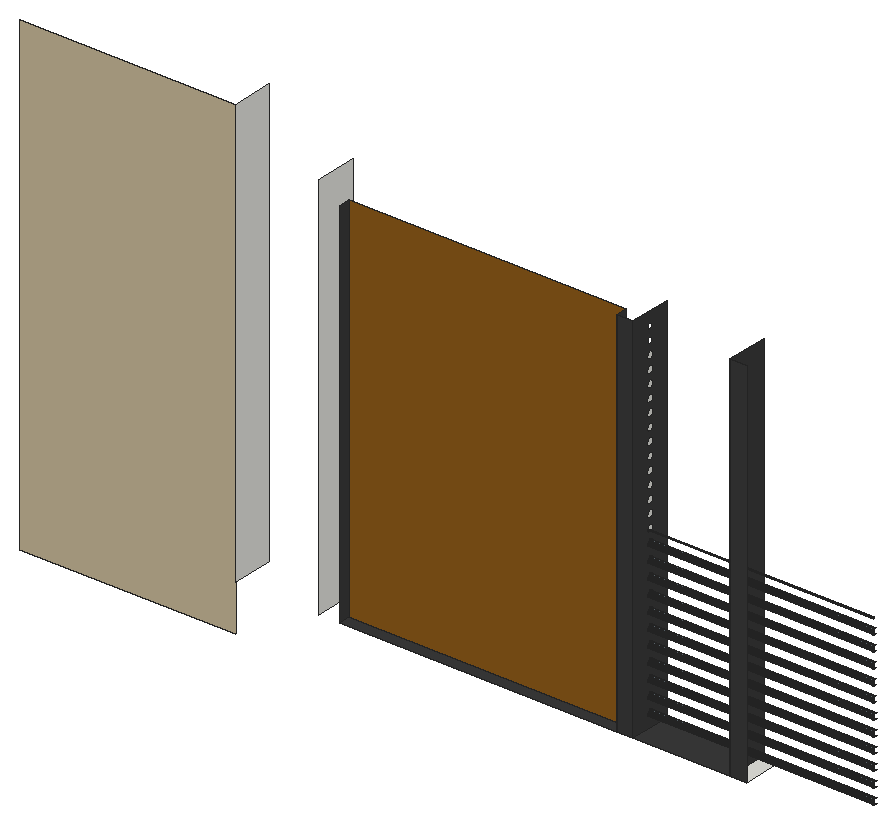
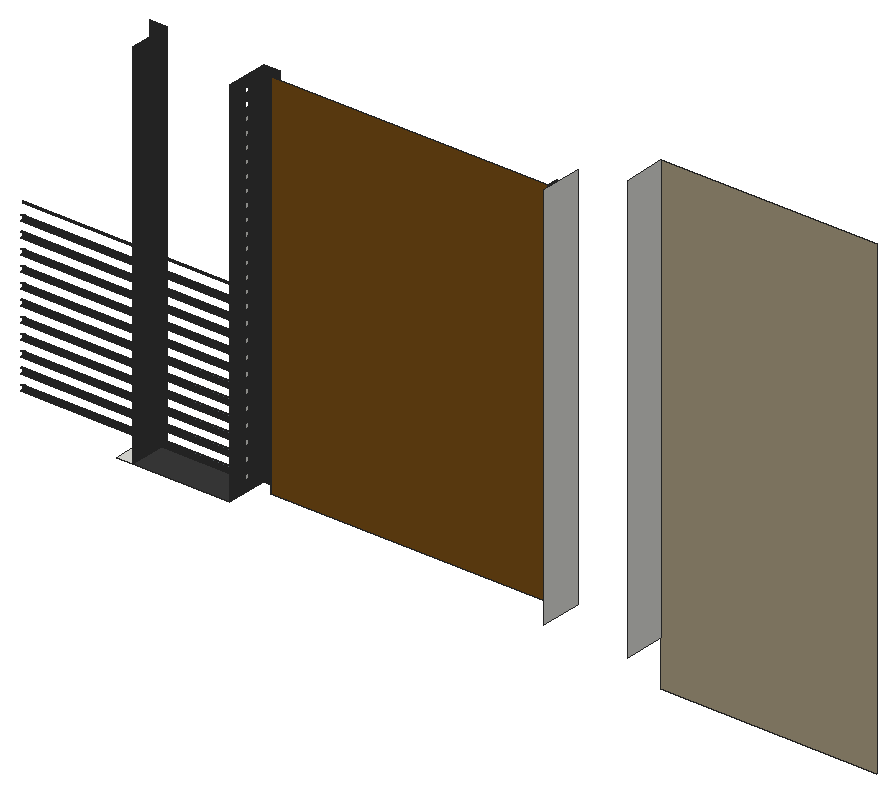
# SketchUp Ruby script. Lengths in inches.
U = 1.inch
M = Sketchup.active_model
def pt(a) = Geom::Point3d.new(a.map { |v| v * U })
def face(e, loops, mat)
  f = e.add_face(loops[0].map { |a| pt(a) })
  loops[1..].each { |l| e.add_face(l.map { |a| pt(a) }).erase! }
  f.material = f.back_material = mat if mat
  f
end
# faces: each face lists its corners as indices into pts; further lists are holes
def faces(e, pts, list, mat = nil) = list.each { |f| face(e, (f[0].is_a?(Array) ? f : [f]).map { |l| l.map { |i| pts[i] } }, mat) }
# xy, xz, yz: faces in a plane at the given z, y or x. An outline is a flat list of corners, or four numbers for a rectangle; further outlines are holes
def ring(l) = l.size == 4 ? [[l[0], l[1]], [l[2], l[1]], [l[2], l[3]], [l[0], l[3]]] : l.each_slice(2).to_a
def flat(e, list, mat, &to3) = list.each { |f| face(e, (f[0].is_a?(Array) ? f : [f]).map { |l| ring(l).map { |u, v| to3.(u, v) } }, mat) }
def xy(e, z, list, mat = nil) = flat(e, list, mat) { |x, y| [x, y, z] }
def xz(e, y, list, mat = nil) = flat(e, list, mat) { |x, z| [x, y, z] }
def yz(e, x, list, mat = nil) = flat(e, list, mat) { |y, z| [x, y, z] }
def lines(e, pts, list) = list.each { |a, b| e.add_line(pt(pts[a]), pt(pts[b])) }
# prism: a flat outline (further loops are holes) pulled along v
def prism(e, loops, v, mat = nil)
  f = face(e, loops, mat); d = Geom::Vector3d.new(v.map { |x| x * U })
  f.pushpull(f.normal.samedirection?(d) ? d.length : -d.length)
end
def box(e, o, s, mat = nil) = prism(e, [[o, [o[0] + s[0], o[1], o[2]], [o[0] + s[0], o[1] + s[1], o[2]], [o[0], o[1] + s[1], o[2]]]], [0, 0, s[2]], mat)
def at(x, y, z, deg = 0) = Geom::Transformation.translation(pt([x, y, z])) * Geom::Transformation.rotation(ORIGIN, Z_AXIS, deg.degrees)
def axes(o, x, y, z) = Geom::Transformation.new([*x, 0, *y, 0, *z, 0, *pt(o).to_a, 1])
def part(name) = M.definitions.add(name)
# library, detail: a bought-in or finely detailed component or shape, given as its bounding box
def library(name, o, s) = part(name).tap { |d| box(d.entities, o, s) }
def detail(e, o, s) = box(e.add_group.entities, o, s)
def put(e, d, t, mat = nil) = e.add_instance(d, t).tap { |i| i.material = mat if mat }
def group(e, t, mat = nil) = e.add_group.tap { |g| g.transformation = t; g.material = mat if mat }.entities
root = M.entities
M.materials.add("[Blinds Weave]").color = [141, 91, 25]
M.materials.add("[Color M07]").color = [58, 58, 58]
M.materials.add("[Formica Speckled Grey]").color = [94, 105, 111]
M.materials.add("[Quartz Light Brown]").color = [199, 184, 152]
xy(root,10.08,[[225.67,279.21,229.25,288.34]])
xy(root,10.08,[[140.74,279.21,201.14,281.7],[204.61,279.21,225.67,288.34]],"[Color M07]")
xz(root,279.21,[[201.14,10.08,204.61,91.34],[225.67,10.08,229.25,91.34]],"[Color M07]")
xz(root,279.21,[[71.32,0,118.15,103.14]],"[Quartz Light Brown]")
xz(root,281.7,[[140.74,10.08,201.14,91.34]],"[Blinds Weave]")
yz(root,118.15,[[279.21,10.08,288.34,103.14]])
yz(root,136.3,[[279.21,10.08,288.34,94.91]])
yz(root,140.74,[[279.21,10.08,281.7,91.34]],"[Color M07]")
yz(root,201.14,[[279.21,10.08,281.7,91.34]],"[Color M07]")
yz(root,204.61,[[283.74,12.45,283.58,12.47,283.43,12.53,283.3,12.63,283.2,12.76,283.14,12.91,283.12,13.07,283.14,13.23,283.2,13.38,283.3,13.51,283.43,13.61,283.58,13.68,283.74,13.7,283.9,13.68,284.05,13.61,284.18,13.51,284.28,13.38,284.34,13.23,284.37,13.07,284.34,12.91,284.28,12.76,284.18,12.63,284.05,12.53,283.9,12.47],[283.74,15.76,283.58,15.78,283.43,15.84,283.3,15.94,283.2,16.07,283.14,16.22,283.12,16.38,283.14,16.55,283.2,16.7,283.3,16.83,283.43,16.93,283.58,16.99,283.74,17.01,283.9,16.99,284.05,16.93,284.18,16.83,284.28,16.7,284.34,16.55,284.37,16.38,284.34,16.22,284.28,16.07,284.18,15.94,284.05,15.84,283.9,15.78],[283.74,19.07,283.58,19.09,283.43,19.16,283.3,19.25,283.2,19.38,283.14,19.54,283.12,19.7,283.14,19.86,283.2,20.01,283.3,20.14,283.43,20.24,283.58,20.3,283.74,20.32,283.9,20.3,284.05,20.24,284.18,20.14,284.28,20.01,284.34,19.86,284.37,19.7,284.34,19.54,284.28,19.38,284.18,19.25,284.05,19.16,283.9,19.09],[283.74,22.38,283.58,22.41,283.43,22.47,283.3,22.57,283.2,22.7,283.14,22.85,283.12,23.01,283.14,23.17,283.2,23.32,283.3,23.45,283.43,23.55,283.58,23.61,283.74,23.63,283.9,23.61,284.05,23.55,284.18,23.45,284.28,23.32,284.34,23.17,284.37,23.01,284.34,22.85,284.28,22.7,284.18,22.57,284.05,22.47,283.9,22.41],[283.74,25.7,283.58,25.72,283.43,25.78,283.3,25.88,283.2,26.01,283.14,26.16,283.12,26.32,283.14,26.48,283.2,26.63,283.3,26.76,283.43,26.86,283.58,26.93,283.74,26.95,283.9,26.93,284.05,26.86,284.18,26.76,284.28,26.63,284.34,26.48,284.37,26.32,284.34,26.16,284.28,26.01,284.18,25.88,284.05,25.78,283.9,25.72],
  [283.74,29.01,283.58,29.03,283.43,29.09,283.3,29.19,283.2,29.32,283.14,29.47,283.12,29.63,283.14,29.8,283.2,29.95,283.3,30.08,283.43,30.18,283.58,30.24,283.74,30.26,283.9,30.24,284.05,30.18,284.18,30.08,284.28,29.95,284.34,29.8,284.37,29.63,284.34,29.47,284.28,29.32,284.18,29.19,284.05,29.09,283.9,29.03],[283.74,32.32,283.58,32.34,283.43,32.41,283.3,32.5,283.2,32.63,283.14,32.79,283.12,32.95,283.14,33.11,283.2,33.26,283.3,33.39,283.43,33.49,283.58,33.55,283.74,33.57,283.9,33.55,284.05,33.49,284.18,33.39,284.28,33.26,284.34,33.11,284.37,32.95,284.34,32.79,284.28,32.63,284.18,32.5,284.05,32.41,283.9,32.34],[283.74,35.63,283.58,35.66,283.43,35.72,283.3,35.82,283.2,35.95,283.14,36.1,283.12,36.26,283.14,36.42,283.2,36.57,283.3,36.7,283.43,36.8,283.58,36.86,283.74,36.88,283.9,36.86,284.05,36.8,284.18,36.7,284.28,36.57,284.34,36.42,284.37,36.26,284.34,36.1,284.28,35.95,284.18,35.82,284.05,35.72,283.9,35.66],[283.74,38.95,283.58,38.97,283.43,39.03,283.3,39.13,283.2,39.26,283.14,39.41,283.12,39.57,283.14,39.73,283.2,39.88,283.3,40.01,283.43,40.11,283.58,40.18,283.74,40.2,283.9,40.18,284.05,40.11,284.18,40.01,284.28,39.88,284.34,39.73,284.37,39.57,284.34,39.41,284.28,39.26,284.18,39.13,284.05,39.03,283.9,38.97],[283.74,42.26,283.58,42.28,283.43,42.34,283.3,42.44,283.2,42.57,283.14,42.72,283.12,42.88,283.14,43.05,283.2,43.2,283.3,43.33,283.43,43.43,283.58,43.49,283.74,43.51,283.9,43.49,284.05,43.43,284.18,43.33,284.28,43.2,284.34,43.05,284.37,42.88,284.34,42.72,284.28,42.57,284.18,42.44,284.05,42.34,283.9,42.28],
  [283.74,45.57,283.58,45.59,283.43,45.66,283.3,45.75,283.2,45.88,283.14,46.04,283.12,46.2,283.14,46.36,283.2,46.51,283.3,46.64,283.43,46.74,283.58,46.8,283.74,46.82,283.9,46.8,284.05,46.74,284.18,46.64,284.28,46.51,284.34,46.36,284.37,46.2,284.34,46.04,284.28,45.88,284.18,45.75,284.05,45.66,283.9,45.59],[283.74,48.38,283.58,48.41,283.43,48.47,283.3,48.57,283.2,48.7,283.14,48.85,283.12,49.01,283.14,49.17,283.2,49.32,283.3,49.45,283.43,49.55,283.58,49.61,283.74,49.63,283.9,49.61,284.05,49.55,284.18,49.45,284.28,49.32,284.34,49.17,284.37,49.01,284.34,48.85,284.28,48.7,284.18,48.57,284.05,48.47,283.9,48.41],[283.74,51.2,283.58,51.22,283.43,51.28,283.3,51.38,283.2,51.51,283.14,51.66,283.12,51.82,283.14,51.98,283.2,52.13,283.3,52.26,283.43,52.36,283.58,52.43,283.74,52.45,283.9,52.43,284.05,52.36,284.18,52.26,284.28,52.13,284.34,51.98,284.37,51.82,284.34,51.66,284.28,51.51,284.18,51.38,284.05,51.28,283.9,51.22],[283.74,54.01,283.58,54.03,283.43,54.09,283.3,54.19,283.2,54.32,283.14,54.47,283.12,54.63,283.14,54.8,283.2,54.95,283.3,55.08,283.43,55.18,283.58,55.24,283.74,55.26,283.9,55.24,284.05,55.18,284.18,55.08,284.28,54.95,284.34,54.8,284.37,54.63,284.34,54.47,284.28,54.32,284.18,54.19,284.05,54.09,283.9,54.03],[283.74,56.82,283.58,56.84,283.43,56.91,283.3,57,283.2,57.13,283.14,57.29,283.12,57.45,283.14,57.61,283.2,57.76,283.3,57.89,283.43,57.99,283.58,58.05,283.74,58.07,283.9,58.05,284.05,57.99,284.18,57.89,284.28,57.76,284.34,57.61,284.37,57.45,284.34,57.29,284.28,57.13,284.18,57,284.05,56.91,283.9,56.84],
  [283.74,59.63,283.58,59.66,283.43,59.72,283.3,59.82,283.2,59.95,283.14,60.1,283.12,60.26,283.14,60.42,283.2,60.57,283.3,60.7,283.43,60.8,283.58,60.86,283.74,60.88,283.9,60.86,284.05,60.8,284.18,60.7,284.28,60.57,284.34,60.42,284.37,60.26,284.34,60.1,284.28,59.95,284.18,59.82,284.05,59.72,283.9,59.66],[283.74,62.45,283.58,62.47,283.43,62.53,283.3,62.63,283.2,62.76,283.14,62.91,283.12,63.07,283.14,63.23,283.2,63.38,283.3,63.51,283.43,63.61,283.58,63.68,283.74,63.7,283.9,63.68,284.05,63.61,284.18,63.51,284.28,63.38,284.34,63.23,284.37,63.07,284.34,62.91,284.28,62.76,284.18,62.63,284.05,62.53,283.9,62.47],[283.74,65.26,283.58,65.28,283.43,65.34,283.3,65.44,283.2,65.57,283.14,65.72,283.12,65.88,283.14,66.05,283.2,66.2,283.3,66.33,283.43,66.43,283.58,66.49,283.74,66.51,283.9,66.49,284.05,66.43,284.18,66.33,284.28,66.2,284.34,66.05,284.37,65.88,284.34,65.72,284.28,65.57,284.18,65.44,284.05,65.34,283.9,65.28],[283.74,68.07,283.58,68.09,283.43,68.16,283.3,68.25,283.2,68.38,283.14,68.54,283.12,68.7,283.14,68.86,283.2,69.01,283.3,69.14,283.43,69.24,283.58,69.3,283.74,69.32,283.9,69.3,284.05,69.24,284.18,69.14,284.28,69.01,284.34,68.86,284.37,68.7,284.34,68.54,284.28,68.38,284.18,68.25,284.05,68.16,283.9,68.09],[283.74,70.88,283.58,70.91,283.43,70.97,283.3,71.07,283.2,71.2,283.14,71.35,283.12,71.51,283.14,71.67,283.2,71.82,283.3,71.95,283.43,72.05,283.58,72.11,283.74,72.13,283.9,72.11,284.05,72.05,284.18,71.95,284.28,71.82,284.34,71.67,284.37,71.51,284.34,71.35,284.28,71.2,284.18,71.07,284.05,70.97,283.9,70.91],
  [283.74,73.7,283.58,73.72,283.43,73.78,283.3,73.88,283.2,74.01,283.14,74.16,283.12,74.32,283.14,74.48,283.2,74.63,283.3,74.76,283.43,74.86,283.58,74.93,283.74,74.95,283.9,74.93,284.05,74.86,284.18,74.76,284.28,74.63,284.34,74.48,284.37,74.32,284.34,74.16,284.28,74.01,284.18,73.88,284.05,73.78,283.9,73.72],[283.74,76.51,283.58,76.53,283.43,76.59,283.3,76.69,283.2,76.82,283.14,76.97,283.12,77.13,283.14,77.3,283.2,77.45,283.3,77.58,283.43,77.68,283.58,77.74,283.74,77.76,283.9,77.74,284.05,77.68,284.18,77.58,284.28,77.45,284.34,77.3,284.37,77.13,284.34,76.97,284.28,76.82,284.18,76.69,284.05,76.59,283.9,76.53],[283.74,79.32,283.58,79.34,283.43,79.41,283.3,79.5,283.2,79.63,283.14,79.79,283.12,79.95,283.14,80.11,283.2,80.26,283.3,80.39,283.43,80.49,283.58,80.55,283.74,80.57,283.9,80.55,284.05,80.49,284.18,80.39,284.28,80.26,284.34,80.11,284.37,79.95,284.34,79.79,284.28,79.63,284.18,79.5,284.05,79.41,283.9,79.34],[283.74,82.13,283.58,82.16,283.43,82.22,283.3,82.32,283.2,82.45,283.14,82.6,283.12,82.76,283.14,82.92,283.2,83.07,283.3,83.2,283.43,83.3,283.58,83.36,283.74,83.38,283.9,83.36,284.05,83.3,284.18,83.2,284.28,83.07,284.34,82.92,284.37,82.76,284.34,82.6,284.28,82.45,284.18,82.32,284.05,82.22,283.9,82.16]])
yz(root,204.61,[[[279.21,10.08,288.34,91.34],[283.74,84.95,283.58,84.97,283.43,85.03,283.3,85.13,283.2,85.26,283.14,85.41,283.12,85.57,283.14,85.73,283.2,85.88,283.3,86.01,283.43,86.11,283.58,86.18,283.74,86.2,283.9,86.18,284.05,86.11,284.18,86.01,284.28,85.88,284.34,85.73,284.37,85.57,284.34,85.41,284.28,85.26,284.18,85.13,284.05,85.03,283.9,84.97],[283.74,82.13,283.58,82.16,283.43,82.22,283.3,82.32,283.2,82.45,283.14,82.6,283.12,82.76,283.14,82.92,283.2,83.07,283.3,83.2,283.43,83.3,283.58,83.36,283.74,83.38,283.9,83.36,284.05,83.3,284.18,83.2,284.28,83.07,284.34,82.92,284.37,82.76,284.34,82.6,284.28,82.45,284.18,82.32,284.05,82.22,283.9,82.16],[283.74,79.32,283.58,79.34,283.43,79.41,283.3,79.5,283.2,79.63,283.14,79.79,283.12,79.95,283.14,80.11,283.2,80.26,283.3,80.39,283.43,80.49,283.58,80.55,283.74,80.57,283.9,80.55,284.05,80.49,284.18,80.39,284.28,80.26,284.34,80.11,284.37,79.95,284.34,79.79,284.28,79.63,284.18,79.5,284.05,79.41,283.9,79.34],[283.74,76.51,283.58,76.53,283.43,76.59,283.3,76.69,283.2,76.82,283.14,76.97,283.12,77.13,283.14,77.3,283.2,77.45,283.3,77.58,283.43,77.68,283.58,77.74,283.74,77.76,283.9,77.74,284.05,77.68,284.18,77.58,284.28,77.45,284.34,77.3,284.37,77.13,284.34,76.97,284.28,76.82,284.18,76.69,284.05,76.59,283.9,76.53],[283.74,73.7,283.58,73.72,283.43,73.78,283.3,73.88,283.2,74.01,283.14,74.16,283.12,74.32,283.14,74.48,283.2,74.63,283.3,74.76,283.43,74.86,283.58,74.93,283.74,74.95,283.9,74.93,284.05,74.86,284.18,74.76,284.28,74.63,284.34,74.48,284.37,74.32,284.34,74.16,284.28,74.01,284.18,73.88,284.05,73.78,283.9,73.72],[283.74,70.88,283.58,70.91,283.43,70.97,283.3,71.07,283.2,71.2,283.14,71.35,283.12,71.51,283.14,71.67,283.2,71.82,283.3,71.95,283.43,72.05,283.58,72.11,283.74,72.13,283.9,72.11,284.05,72.05,284.18,71.95,284.28,71.82,284.34,71.67,284.37,71.51,284.34,71.35,284.28,71.2,284.18,71.07,284.05,70.97,283.9,70.91],[283.74,68.07,283.58,68.09,283.43,68.16,283.3,68.25,283.2,68.38,283.14,68.54,283.12,68.7,283.14,68.86,283.2,69.01,283.3,69.14,283.43,69.24,283.58,69.3,283.74,69.32,283.9,69.3,284.05,69.24,284.18,69.14,284.28,69.01,284.34,68.86,284.37,68.7,284.34,68.54,284.28,68.38,284.18,68.25,284.05,68.16,283.9,68.09],[283.74,65.26,283.58,65.28,283.43,65.34,283.3,65.44,283.2,65.57,283.14,65.72,283.12,65.88,283.14,66.05,283.2,66.2,283.3,66.33,283.43,66.43,283.58,66.49,283.74,66.51,283.9,66.49,284.05,66.43,284.18,66.33,284.28,66.2,284.34,66.05,284.37,65.88,284.34,65.72,284.28,65.57,284.18,65.44,284.05,65.34,283.9,65.28],[283.74,62.45,283.58,62.47,283.43,62.53,283.3,62.63,283.2,62.76,283.14,62.91,283.12,63.07,283.14,63.23,283.2,63.38,283.3,63.51,283.43,63.61,283.58,63.68,283.74,63.7,283.9,63.68,284.05,63.61,284.18,63.51,284.28,63.38,284.34,63.23,284.37,63.07,284.34,62.91,284.28,62.76,284.18,62.63,284.05,62.53,283.9,62.47],[283.74,59.63,283.58,59.66,283.43,59.72,283.3,59.82,283.2,59.95,283.14,60.1,283.12,60.26,283.14,60.42,283.2,60.57,283.3,60.7,283.43,60.8,283.58,60.86,283.74,60.88,283.9,60.86,284.05,60.8,284.18,60.7,284.28,60.57,284.34,60.42,284.37,60.26,284.34,60.1,284.28,59.95,284.18,59.82,284.05,59.72,283.9,59.66],[283.74,56.82,283.58,56.84,283.43,56.91,283.3,57,283.2,57.13,283.14,57.29,283.12,57.45,283.14,57.61,283.2,57.76,283.3,57.89,283.43,57.99,283.58,58.05,283.74,58.07,283.9,58.05,284.05,57.99,284.18,57.89,284.28,57.76,284.34,57.61,284.37,57.45,284.34,57.29,284.28,57.13,284.18,57,284.05,56.91,283.9,56.84],[283.74,54.01,283.58,54.03,283.43,54.09,283.3,54.19,283.2,54.32,283.14,54.47,283.12,54.63,283.14,54.8,283.2,54.95,283.3,55.08,283.43,55.18,283.58,55.24,283.74,55.26,283.9,55.24,284.05,55.18,284.18,55.08,284.28,54.95,284.34,54.8,284.37,54.63,284.34,54.47,284.28,54.32,284.18,54.19,284.05,54.09,283.9,54.03],[283.74,51.2,283.58,51.22,283.43,51.28,283.3,51.38,283.2,51.51,283.14,51.66,283.12,51.82,283.14,51.98,283.2,52.13,283.3,52.26,283.43,52.36,283.58,52.43,283.74,52.45,283.9,52.43,284.05,52.36,284.18,52.26,284.28,52.13,284.34,51.98,284.37,51.82,284.34,51.66,284.28,51.51,284.18,51.38,284.05,51.28,283.9,51.22],[283.74,48.38,283.58,48.41,283.43,48.47,283.3,48.57,283.2,48.7,283.14,48.85,283.12,49.01,283.14,49.17,283.2,49.32,283.3,49.45,283.43,49.55,283.58,49.61,283.74,49.63,283.9,49.61,284.05,49.55,284.18,49.45,284.28,49.32,284.34,49.17,284.37,49.01,284.34,48.85,284.28,48.7,284.18,48.57,284.05,48.47,283.9,48.41],[283.74,45.57,283.58,45.59,283.43,45.66,283.3,45.75,283.2,45.88,283.14,46.04,283.12,46.2,283.14,46.36,283.2,46.51,283.3,46.64,283.43,46.74,283.58,46.8,283.74,46.82,283.9,46.8,284.05,46.74,284.18,46.64,284.28,46.51,284.34,46.36,284.37,46.2,284.34,46.04,284.28,45.88,284.18,45.75,284.05,45.66,283.9,45.59],[283.74,42.26,283.58,42.28,283.43,42.34,283.3,42.44,283.2,42.57,283.14,42.72,283.12,42.88,283.14,43.05,283.2,43.2,283.3,43.33,283.43,43.43,283.58,43.49,283.74,43.51,283.9,43.49,284.05,43.43,284.18,43.33,284.28,43.2,284.34,43.05,284.37,42.88,284.34,42.72,284.28,42.57,284.18,42.44,284.05,42.34,283.9,42.28],[283.74,38.95,283.58,38.97,283.43,39.03,283.3,39.13,283.2,39.26,283.14,39.41,283.12,39.57,283.14,39.73,283.2,39.88,283.3,40.01,283.43,40.11,283.58,40.18,283.74,40.2,283.9,40.18,284.05,40.11,284.18,40.01,284.28,39.88,284.34,39.73,284.37,39.57,284.34,39.41,284.28,39.26,284.18,39.13,284.05,39.03,283.9,38.97],[283.74,35.63,283.58,35.66,283.43,35.72,283.3,35.82,283.2,35.95,283.14,36.1,283.12,36.26,283.14,36.42,283.2,36.57,283.3,36.7,283.43,36.8,283.58,36.86,283.74,36.88,283.9,36.86,284.05,36.8,284.18,36.7,284.28,36.57,284.34,36.42,284.37,36.26,284.34,36.1,284.28,35.95,284.18,35.82,284.05,35.72,283.9,35.66],[283.74,32.32,283.58,32.34,283.43,32.41,283.3,32.5,283.2,32.63,283.14,32.79,283.12,32.95,283.14,33.11,283.2,33.26,283.3,33.39,283.43,33.49,283.58,33.55,283.74,33.57,283.9,33.55,284.05,33.49,284.18,33.39,284.28,33.26,284.34,33.11,284.37,32.95,284.34,32.79,284.28,32.63,284.18,32.5,284.05,32.41,283.9,32.34],[283.74,29.01,283.58,29.03,283.43,29.09,283.3,29.19,283.2,29.32,283.14,29.47,283.12,29.63,283.14,29.8,283.2,29.95,283.3,30.08,283.43,30.18,283.58,30.24,283.74,30.26,283.9,30.24,284.05,30.18,284.18,30.08,284.28,29.95,284.34,29.8,284.37,29.63,284.34,29.47,284.28,29.32,284.18,29.19,284.05,29.09,283.9,29.03],[283.74,25.7,283.58,25.72,283.43,25.78,283.3,25.88,283.2,26.01,283.14,26.16,283.12,26.32,283.14,26.48,283.2,26.63,283.3,26.76,283.43,26.86,283.58,26.93,283.74,26.95,283.9,26.93,284.05,26.86,284.18,26.76,284.28,26.63,284.34,26.48,284.37,26.32,284.34,26.16,284.28,26.01,284.18,25.88,284.05,25.78,283.9,25.72],[283.74,22.38,283.58,22.41,283.43,22.47,283.3,22.57,283.2,22.7,283.14,22.85,283.12,23.01,283.14,23.17,283.2,23.32,283.3,23.45,283.43,23.55,283.58,23.61,283.74,23.63,283.9,23.61,284.05,23.55,284.18,23.45,284.28,23.32,284.34,23.17,284.37,23.01,284.34,22.85,284.28,22.7,284.18,22.57,284.05,22.47,283.9,22.41],[283.74,19.07,283.58,19.09,283.43,19.16,283.3,19.25,283.2,19.38,283.14,19.54,283.12,19.7,283.14,19.86,283.2,20.01,283.3,20.14,283.43,20.24,283.58,20.3,283.74,20.32,283.9,20.3,284.05,20.24,284.18,20.14,284.28,20.01,284.34,19.86,284.37,19.7,284.34,19.54,284.28,19.38,284.18,19.25,284.05,19.16,283.9,19.09],[283.74,15.76,283.58,15.78,283.43,15.84,283.3,15.94,283.2,16.07,283.14,16.22,283.12,16.38,283.14,16.55,283.2,16.7,283.3,16.83,283.43,16.93,283.58,16.99,283.74,17.01,283.9,16.99,284.05,16.93,284.18,16.83,284.28,16.7,284.34,16.55,284.37,16.38,284.34,16.22,284.28,16.07,284.18,15.94,284.05,15.84,283.9,15.78],[283.74,12.45,283.58,12.47,283.43,12.53,283.3,12.63,283.2,12.76,283.14,12.91,283.12,13.07,283.14,13.23,283.2,13.38,283.3,13.51,283.43,13.61,283.58,13.68,283.74,13.7,283.9,13.68,284.05,13.61,284.18,13.51,284.28,13.38,284.34,13.23,284.37,13.07,284.34,12.91,284.28,12.76,284.18,12.63,284.05,12.53,283.9,12.47],[283.74,87.76,283.58,87.78,283.43,87.84,283.3,87.94,283.2,88.07,283.14,88.22,283.12,88.38,283.14,88.55,283.2,88.7,283.3,88.83,283.43,88.93,283.58,88.99,283.74,89.01,283.9,88.99,284.05,88.93,284.18,88.83,284.28,88.7,284.34,88.55,284.37,88.38,284.34,88.22,284.28,88.07,284.18,87.94,284.05,87.84,283.9,87.78]]],"[Color M07]")
yz(root,225.67,[[279.21,10.08,288.34,91.34]],"[Color M07]")
p = [[204.61,283.58,12.47],[204.61,283.74,12.45],[253.76,283.74,12.45],[253.76,283.58,12.47],[204.61,283.9,12.47],[253.76,283.9,12.47],
  [204.61,283.3,12.63],[204.61,283.43,12.53],[253.76,283.43,12.53],[253.76,283.3,12.63],[204.61,283.2,12.76],[253.76,283.2,12.76],
  [204.61,283.14,12.91],[253.76,283.14,12.91],[204.61,283.12,13.07],[253.76,283.12,13.07],[204.61,283.14,13.23],[253.76,283.14,13.23],
  [204.61,283.2,13.38],[253.76,283.2,13.38],[204.61,283.3,13.51],[253.76,283.3,13.51],[204.61,283.43,13.61],[253.76,283.43,13.61],
  [204.61,283.58,13.68],[253.76,283.58,13.68],[204.61,283.74,13.7],[253.76,283.74,13.7],[204.61,283.9,13.68],[253.76,283.9,13.68],
  [204.61,283.3,15.94],[204.61,283.43,15.84],[253.76,283.43,15.84],[253.76,283.3,15.94],[204.61,283.58,15.78],[253.76,283.58,15.78],
  [204.61,283.74,15.76],[253.76,283.74,15.76],[204.61,283.9,15.78],[253.76,283.9,15.78],[204.61,283.2,16.07],[253.76,283.2,16.07],
  [204.61,283.14,16.22],[253.76,283.14,16.22],[204.61,283.12,16.38],[253.76,283.12,16.38],[204.61,283.14,16.55],[253.76,283.14,16.55],
  [204.61,283.2,16.7],[253.76,283.2,16.7],[204.61,283.3,16.83],[253.76,283.3,16.83],[204.61,283.43,16.93],[253.76,283.43,16.93],
  [204.61,283.58,16.99],[253.76,283.58,16.99],[204.61,283.74,17.01],[253.76,283.74,17.01],[204.61,283.9,16.99],[253.76,283.9,16.99],
  [204.61,283.43,19.16],[204.61,283.58,19.09],[253.76,283.58,19.09],[253.76,283.43,19.16],[204.61,283.74,19.07],[253.76,283.74,19.07],
  [204.61,283.9,19.09],[253.76,283.9,19.09],[204.61,283.3,19.25],[253.76,283.3,19.25],[204.61,283.2,19.38],[253.76,283.2,19.38],
  [204.61,283.14,19.54],[253.76,283.14,19.54],[204.61,283.12,19.7],[253.76,283.12,19.7],[204.61,283.14,19.86],[253.76,283.14,19.86],
  [204.61,283.2,20.01],[253.76,283.2,20.01],[204.61,283.3,20.14],[253.76,283.3,20.14],[204.61,283.43,20.24],[253.76,283.43,20.24],
  [204.61,283.58,20.3],[253.76,283.58,20.3],[204.61,283.74,20.32],[253.76,283.74,20.32],[204.61,283.9,20.3],[253.76,283.9,20.3],
  [204.61,283.43,22.47],[204.61,283.58,22.41],[253.76,283.58,22.41],[253.76,283.43,22.47],[204.61,283.74,22.38],[253.76,283.74,22.38],
  [204.61,283.9,22.41],[253.76,283.9,22.41],[204.61,283.3,22.57],[253.76,283.3,22.57],[204.61,283.2,22.7],[253.76,283.2,22.7],
  [204.61,283.14,22.85],[253.76,283.14,22.85],[204.61,283.12,23.01],[253.76,283.12,23.01],[204.61,283.14,23.17],[253.76,283.14,23.17],
  [204.61,283.2,23.32],[253.76,283.2,23.32],[204.61,283.3,23.45],[253.76,283.3,23.45],[204.61,283.43,23.55],[253.76,283.43,23.55],
  [204.61,283.58,23.61],[253.76,283.58,23.61],[204.61,283.74,23.63],[253.76,283.74,23.63],[204.61,283.9,23.61],[253.76,283.9,23.61],
  [204.61,283.43,25.78],[204.61,283.58,25.72],[253.76,283.58,25.72],[253.76,283.43,25.78],[204.61,283.74,25.7],[253.76,283.74,25.7],
  [204.61,283.9,25.72],[253.76,283.9,25.72],[204.61,283.3,25.88],[253.76,283.3,25.88],[204.61,283.2,26.01],[253.76,283.2,26.01],
  [204.61,283.14,26.16],[253.76,283.14,26.16],[204.61,283.12,26.32],[253.76,283.12,26.32],[204.61,283.14,26.48],[253.76,283.14,26.48],
  [204.61,283.2,26.63],[253.76,283.2,26.63],[204.61,283.3,26.76],[253.76,283.3,26.76],[204.61,283.43,26.86],[253.76,283.43,26.86],
  [204.61,283.58,26.93],[253.76,283.58,26.93],[204.61,283.74,26.95],[253.76,283.74,26.95],[204.61,283.9,26.93],[253.76,283.9,26.93],
  [204.61,283.43,29.09],[204.61,283.58,29.03],[253.76,283.58,29.03],[253.76,283.43,29.09],[204.61,283.74,29.01],[253.76,283.74,29.01],
  [204.61,283.9,29.03],[253.76,283.9,29.03],[204.61,283.3,29.19],[253.76,283.3,29.19],[204.61,283.2,29.32],[253.76,283.2,29.32],
  [204.61,283.14,29.47],[253.76,283.14,29.47],[204.61,283.12,29.63],[253.76,283.12,29.63],[204.61,283.14,29.8],[253.76,283.14,29.8],
  [204.61,283.2,29.95],[253.76,283.2,29.95],[204.61,283.3,30.08],[253.76,283.3,30.08],[204.61,283.43,30.18],[253.76,283.43,30.18],
  [204.61,283.58,30.24],[253.76,283.58,30.24],[204.61,283.74,30.26],[253.76,283.74,30.26],[204.61,283.9,30.24],[253.76,283.9,30.24],
  [204.61,283.43,32.41],[204.61,283.58,32.34],[253.76,283.58,32.34],[253.76,283.43,32.41],[204.61,283.74,32.32],[253.76,283.74,32.32],
  [204.61,283.3,32.5],[253.76,283.3,32.5],[204.61,283.2,32.63],[253.76,283.2,32.63],[204.61,283.14,32.79],[253.76,283.14,32.79],
  [204.61,283.12,32.95],[253.76,283.12,32.95],[204.61,283.14,33.11],[253.76,283.14,33.11],[204.61,283.2,33.26],[253.76,283.2,33.26],
  [204.61,283.3,33.39],[253.76,283.3,33.39],[204.61,283.43,33.49],[253.76,283.43,33.49],[204.61,283.58,33.55],[253.76,283.58,33.55],
  [204.61,283.74,33.57],[253.76,283.74,33.57],[204.61,283.58,35.66],[204.61,283.74,35.63],[253.76,283.74,35.63],[253.76,283.58,35.66],
  [204.61,283.3,35.82],[204.61,283.43,35.72],[253.76,283.43,35.72],[253.76,283.3,35.82],[204.61,283.2,35.95],[253.76,283.2,35.95],
  [204.61,283.14,36.1],[253.76,283.14,36.1],[204.61,283.12,36.26],[253.76,283.12,36.26],[204.61,283.14,36.42],[253.76,283.14,36.42],
  [204.61,283.2,36.57],[253.76,283.2,36.57],[204.61,283.3,36.7],[253.76,283.3,36.7],[204.61,283.43,36.8],[253.76,283.43,36.8],
  [204.61,283.58,36.86],[253.76,283.58,36.86],[204.61,283.74,36.88],[253.76,283.74,36.88],[204.61,283.58,38.97],[204.61,283.74,38.95],
  [253.76,283.74,38.95],[253.76,283.58,38.97],[204.61,283.3,39.13],[204.61,283.43,39.03],[253.76,283.43,39.03],[253.76,283.3,39.13],
  [204.61,283.2,39.26],[253.76,283.2,39.26],[204.61,283.14,39.41],[253.76,283.14,39.41],[204.61,283.12,39.57],[253.76,283.12,39.57],
  [204.61,283.14,39.73],[253.76,283.14,39.73],[204.61,283.2,39.88],[253.76,283.2,39.88],[204.61,283.3,40.01],[253.76,283.3,40.01],
  [204.61,283.43,40.11],[253.76,283.43,40.11],[204.61,283.58,40.18],[253.76,283.58,40.18],[204.61,283.74,40.2],[253.76,283.74,40.2],
  [204.61,283.3,42.44],[204.61,283.43,42.34],[253.76,283.43,42.34],[253.76,283.3,42.44],[204.61,283.58,42.28],[253.76,283.58,42.28],
  [204.61,283.74,42.26],[253.76,283.74,42.26],[204.61,283.2,42.57],[253.76,283.2,42.57],[204.61,283.14,42.72],[253.76,283.14,42.72],
  [204.61,283.12,42.88],[253.76,283.12,42.88],[204.61,283.14,43.05],[253.76,283.14,43.05],[204.61,283.2,43.2],[253.76,283.2,43.2],
  [204.61,283.3,43.33],[253.76,283.3,43.33],[204.61,283.43,43.43],[253.76,283.43,43.43],[204.61,283.58,43.49],[253.76,283.58,43.49],
  [204.61,283.74,43.51],[253.76,283.74,43.51],[204.61,283.43,45.66],[204.61,283.58,45.59],[253.76,283.58,45.59],[253.76,283.43,45.66],
  [204.61,283.74,45.57],[253.76,283.74,45.57],[204.61,283.3,45.75],[253.76,283.3,45.75],[204.61,283.2,45.88],[253.76,283.2,45.88],
  [204.61,283.14,46.04],[253.76,283.14,46.04],[204.61,283.12,46.2],[253.76,283.12,46.2],[204.61,283.14,46.36],[253.76,283.14,46.36],
  [204.61,283.2,46.51],[253.76,283.2,46.51],[204.61,283.3,46.64],[253.76,283.3,46.64],[204.61,283.43,46.74],[253.76,283.43,46.74],
  [204.61,283.58,46.8],[253.76,283.58,46.8],[204.61,283.74,46.82],[253.76,283.74,46.82],[204.61,283.12,49.01],[204.61,283.14,48.85],
  [253.76,283.14,48.85],[253.76,283.12,49.01],[204.61,283.14,49.17],[253.76,283.14,49.17]]
faces(root,p,[[0,1,2,3],[1,4,5,2],[6,7,8,9],[7,0,3,8],[10,6,9,11],[12,10,11,13],[14,12,13,15],[16,14,15,17],
  [18,16,17,19],[20,18,19,21],[22,20,21,23],[24,22,23,25],[26,24,25,27],[28,26,27,29],[30,31,32,33],[31,34,35,32],
  [34,36,37,35],[36,38,39,37],[40,30,33,41],[42,40,41,43],[44,42,43,45],[46,44,45,47],[48,46,47,49],[50,48,49,51],
  [52,50,51,53],[54,52,53,55],[56,54,55,57],[58,56,57,59],[60,61,62,63],[61,64,65,62],[64,66,67,65],[68,60,63,69],
  [70,68,69,71],[72,70,71,73],[74,72,73,75],[76,74,75,77],[78,76,77,79],[80,78,79,81],[82,80,81,83],[84,82,83,85],
  [86,84,85,87],[88,86,87,89],[90,91,92,93],[91,94,95,92],[94,96,97,95],[98,90,93,99],[100,98,99,101],[102,100,101,103],
  [104,102,103,105],[106,104,105,107],[108,106,107,109],[110,108,109,111],[112,110,111,113],[114,112,113,115],[116,114,115,117],[118,116,117,119],
  [120,121,122,123],[121,124,125,122],[124,126,127,125],[128,120,123,129],[130,128,129,131],[132,130,131,133],[134,132,133,135],[136,134,135,137],
  [138,136,137,139],[140,138,139,141],[142,140,141,143],[144,142,143,145],[146,144,145,147],[148,146,147,149],[150,151,152,153],[151,154,155,152],
  [154,156,157,155],[158,150,153,159],[160,158,159,161],[162,160,161,163],[164,162,163,165],[166,164,165,167],[168,166,167,169],[170,168,169,171],
  [172,170,171,173],[174,172,173,175],[176,174,175,177],[178,176,177,179],[180,181,182,183],[181,184,185,182],[186,180,183,187],[188,186,187,189],
  [190,188,189,191],[192,190,191,193],[194,192,193,195],[196,194,195,197],[198,196,197,199],[200,198,199,201],[202,200,201,203],[204,202,203,205],
  [206,207,208,209],[210,211,212,213],[211,206,209,212],[214,210,213,215],[216,214,215,217],[218,216,217,219],[220,218,219,221],[222,220,221,223],
  [224,222,223,225],[226,224,225,227],[228,226,227,229],[230,228,229,231],[232,233,234,235],[236,237,238,239],[237,232,235,238],[240,236,239,241],
  [242,240,241,243],[244,242,243,245],[246,244,245,247],[248,246,247,249],[250,248,249,251],[252,250,251,253],[254,252,253,255],[256,254,255,257],
  [258,259,260,261],[259,262,263,260],[262,264,265,263],[266,258,261,267],[268,266,267,269],[270,268,269,271],[272,270,271,273],[274,272,273,275],
  [276,274,275,277],[278,276,277,279],[280,278,279,281],[282,280,281,283],[284,285,286,287],[285,288,289,286],[290,284,287,291],[292,290,291,293],
  [294,292,293,295],[296,294,295,297],[298,296,297,299],[300,298,299,301],[302,300,301,303],[304,302,303,305],[306,304,305,307],[308,306,307,309],
  [310,311,312,313],[314,310,313,315]],"[Formica Speckled Grey]")
